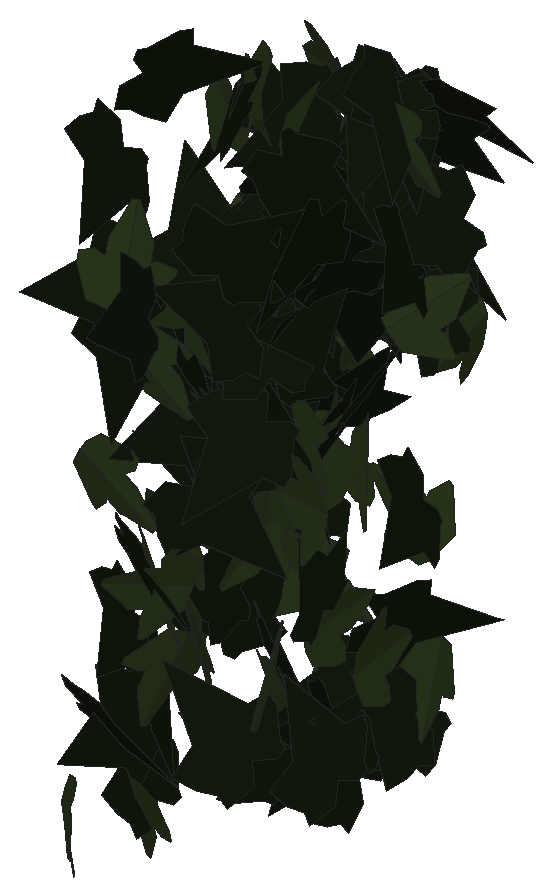
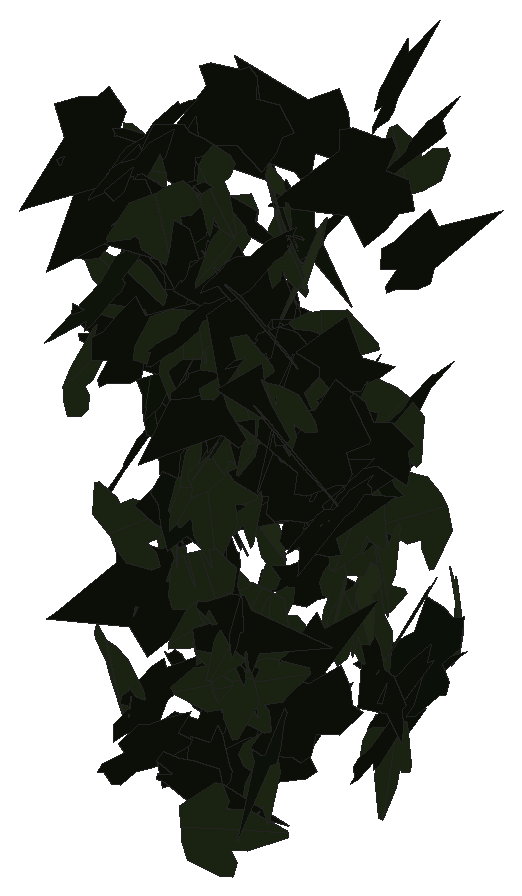
# SketchUp Ruby script. Lengths in inches.
U = 1.inch
M = Sketchup.active_model
def pt(a) = Geom::Point3d.new(a.map { |v| v * U })
def face(e, loops, mat)
  f = e.add_face(loops[0].map { |a| pt(a) })
  loops[1..].each { |l| e.add_face(l.map { |a| pt(a) }).erase! }
  f.material = f.back_material = mat if mat
  f
end
# faces: each face lists its corners as indices into pts; further lists are holes
def faces(e, pts, list, mat = nil) = list.each { |f| face(e, (f[0].is_a?(Array) ? f : [f]).map { |l| l.map { |i| pts[i] } }, mat) }
# xy, xz, yz: faces in a plane at the given z, y or x. An outline is a flat list of corners, or four numbers for a rectangle; further outlines are holes
def ring(l) = l.size == 4 ? [[l[0], l[1]], [l[2], l[1]], [l[2], l[3]], [l[0], l[3]]] : l.each_slice(2).to_a
def flat(e, list, mat, &to3) = list.each { |f| face(e, (f[0].is_a?(Array) ? f : [f]).map { |l| ring(l).map { |u, v| to3.(u, v) } }, mat) }
def xy(e, z, list, mat = nil) = flat(e, list, mat) { |x, y| [x, y, z] }
def xz(e, y, list, mat = nil) = flat(e, list, mat) { |x, z| [x, y, z] }
def yz(e, x, list, mat = nil) = flat(e, list, mat) { |y, z| [x, y, z] }
def lines(e, pts, list) = list.each { |a, b| e.add_line(pt(pts[a]), pt(pts[b])) }
# prism: a flat outline (further loops are holes) pulled along v
def prism(e, loops, v, mat = nil)
  f = face(e, loops, mat); d = Geom::Vector3d.new(v.map { |x| x * U })
  f.pushpull(f.normal.samedirection?(d) ? d.length : -d.length)
end
def box(e, o, s, mat = nil) = prism(e, [[o, [o[0] + s[0], o[1], o[2]], [o[0] + s[0], o[1] + s[1], o[2]], [o[0], o[1] + s[1], o[2]]]], [0, 0, s[2]], mat)
def at(x, y, z, deg = 0) = Geom::Transformation.translation(pt([x, y, z])) * Geom::Transformation.rotation(ORIGIN, Z_AXIS, deg.degrees)
def axes(o, x, y, z) = Geom::Transformation.new([*x, 0, *y, 0, *z, 0, *pt(o).to_a, 1])
def part(name) = M.definitions.add(name)
# library, detail: a bought-in or finely detailed component or shape, given as its bounding box
def library(name, o, s) = part(name).tap { |d| box(d.entities, o, s) }
def detail(e, o, s) = box(e.add_group.entities, o, s)
def put(e, d, t, mat = nil) = e.add_instance(d, t).tap { |i| i.material = mat if mat }
def group(e, t, mat = nil) = e.add_group.tap { |g| g.transformation = t; g.material = mat if mat }.entities
root = M.entities
M.materials.add("efeu1").color = [18, 25, 13]
M.materials.add("efeu2").color = [43, 57, 29]
c1 = part("ivyleaf_9")
p = [[1.54,2.16,1.25],[1.36,2.04,1.19],[-0.21,0.99,0.68],[-0.71,1.11,0.82],[-0.85,0.86,0.67],[-0.8,0.17,0.21],
  [-0.9,-0.01,0.1],[-0.67,-0.16,-0.02],[-0.08,-0.08,-0.05],[-0.03,-0.6,-0.4],[0.65,-0.88,-0.66],[0.83,-0.6,-0.49],
  [1.29,-0.42,-0.43],[1.8125,-0.07,-0.26],[1.21,0.44,0.15]]
faces(c1.entities,p,[[0,1,2,3,4,5,6,7,8,9,10,11,12,13,14]],"efeu1")
c2 = part("ivyleaf_10")
p = [[0,0.5,-0.03],[-0.0625,2.02,-0.43],[-0.19,2.01,-0.46],[-0.54,1.05,-0.29],[-0.52,0.625,-0.18],[-0.83,0.76,-0.28],
  [-1.16,0.64,-0.33],[-1.15,0.33,-0.24],[-0.77,-0.39,0.02],[-0.3,-0.51,0.16],[0.04,-0.48,0.23],[-0.02,2.01,-0.4375],
  [-0.06,2.01,-0.43],[0.04,-0.49,0.23],[0.67,-0.49,0.14],[1.38,0.36,-0.2],[1.375,0.51,-0.24],[0.81,0.65,-0.19],
  [0.62,0.59,-0.15],[0.6,1.09,-0.28],[0.5,1.23,-0.31]]
faces(c2.entities,p,[[0,1,2,3,4,5,6,7,8,9,10],[11,12,0,13,14,15,16,17,18,19,20]],"efeu2")
put(root,c1,axes([52.25,217.93,221.68],[-0.05075,-0.13699,0.47818],[-0.12594,-0.46146,-0.14557],[0.48121,-0.13522,0.01233]))
put(root,c2,axes([51.13,217.92,214.84],[-0.0102,0.01905,-0.49953],[0.22698,-0.44499,-0.0216],[-0.44539,-0.22721,0.00043]))
put(root,c2,axes([51.17,218.83,221.32],[0.2368,0.40848,-0.16453],[0.08062,0.14344,0.47215],[0.43293,-0.25014,0.00207]))
put(root,c1,axes([52.59,219.37,215.44],[-0.32768,-0.37509,-0.04394],[-0.02902,-0.03299,0.49807],[-0.37654,0.32896,-0.00015]))
put(root,c1,axes([50.58,219.68,220.76],[-0.1492,-0.11801,0.4624],[-0.32053,-0.33415,-0.1887],[0.35355,-0.35273,0.02406]))
put(root,c1,axes([50.24,219.4,215.24],[0.36828,-0.22379,0.25354],[0.22278,-0.12149,-0.43083],[0.25443,0.4303,0.01023]))
put(root,c1,axes([50.43,219.76,222.44],[-0.05996,-0.41817,0.26747],[-0.03648,-0.26497,-0.42245],[0.49505,-0.07018,0.00126]))
put(root,c1,axes([52.24,219.35,221.66],[-0.1215,-0.01743,0.4847],[0.46596,-0.14288,0.11166],[0.13462,0.47883,0.05096]))
put(root,c1,axes([50.73,219.52,217.54],[0.43208,-0.20442,-0.14669],[-0.13039,0.06738,-0.47797],[0.21519,0.4513,0.00491]))
put(root,c2,axes([51.09,219.95,216.88],[-0.14081,-0.09889,-0.46946],[-0.26462,-0.3921,0.16197],[-0.40018,0.29407,0.05809]))
put(root,c1,axes([50.5,220.03,214.89],[-0.14103,-0.24196,0.41421],[-0.17159,-0.37773,-0.27907],[0.44796,-0.22086,0.0235]))
put(root,c2,axes([52.625,219.58,216],[0.23907,-0.31924,0.30155],[-0.18248,0.24007,0.39883],[-0.39943,-0.30075,-0.00172]))
put(root,c1,axes([51.95,220.09,220.54],[0.05866,-0.47673,-0.13887],[0.01816,-0.13768,0.48033],[-0.49621,-0.0614,0.00116]))
put(root,c2,axes([50.73,219.71,214.18],[-0.44327,0.19916,0.11769],[-0.10581,0.05164,-0.48594],[-0.20572,-0.45571,-0.00363]))
put(root,c2,axes([51,220.08,215.98],[-0.08545,-0.45152,0.19705],[-0.01764,-0.19706,-0.45919],[0.49233,-0.08543,0.01774]))
put(root,c1,axes([50.12,220.36,216],[-0.03885,-0.30869,0.39141],[0.00307,-0.39274,-0.30943],[0.49848,-0.02163,0.03241]))
put(root,c1,axes([50.73,220,214.01],[-0.12055,-0.43794,0.20899],[0.06163,0.19978,0.45419],[-0.48132,0.13526,0.00581]))
put(root,c1,axes([53,220.18,222.23],[-0.0923,0.2247,-0.43702],[0.18885,-0.3943,-0.24262],[-0.45367,-0.20985,-0.01208]))
put(root,c1,axes([51.35,219.98,218.21],[-0.0338,-0.1462,-0.47695],[0.19794,0.43487,-0.14733],[0.4579,-0.19878,0.02848]))
put(root,c2,axes([49.74,220.21,217.9],[-0.27428,0.08199,-0.40994],[0.38793,-0.13282,-0.28612],[-0.15581,-0.47501,0.00925]))
put(root,c1,axes([50.33,220.36,215.52],[-0.15855,-0.03336,-0.47302],[0.47069,0.04945,-0.16126],[0.05754,-0.49643,0.01572]))
put(root,c2,axes([51.19,220.17,216.31],[-0.34414,0.36112,-0.03405],[0.02139,-0.02665,-0.49883],[-0.36209,-0.34479,0.0029]))
put(root,c2,axes([50.18,220.46,216.85],[-0.11885,0.0154,0.48542],[0.42602,-0.23666,0.11181],[0.2332,0.44018,0.04314]))
put(root,c2,axes([50.84,220.2,217.64],[-0.48213,0.1028,-0.08356],[0.08293,-0.01175,-0.49293],[-0.10332,-0.48918,-0.00572]))
put(root,c1,axes([51.88,220.52,219.03],[-0.44839,-0.22096,0.01116],[-0.00958,-0.0058,-0.49987],[0.22103,-0.44849,0.00097]))
put(root,c2,axes([52.94,220.13,218.47],[0.10992,-0.10806,-0.47565],[-0.36318,0.30734,-0.15375],[0.3256,0.37929,-0.01092]))
put(root,c1,axes([49.8,220.63,219.45],[0.01371,-0.47099,0.16728],[0.00304,-0.16727,-0.47118],[0.4998,0.01394,-0.00172]))
put(root,c2,axes([50.93,220.04,216.19],[0.12633,0.06004,-0.48004],[-0.26803,0.42172,-0.01779],[0.40274,0.26182,0.13874]))
put(root,c1,axes([52.35,220.375,222.72],[-0.02827,-0.02411,-0.49862],[0.33873,0.36592,-0.0369],[0.36669,-0.33988,-0.00435]))
put(root,c1,axes([53.03,220.42,214.88],[-0.4542,-0.02889,-0.20704],[-0.20675,-0.01123,0.45512],[-0.03094,0.49904,-0.00174]))
put(root,c1,axes([52.08,220.43,219.82],[-0.48137,-0.02435,0.13301],[0.13306,0.00211,0.48196],[-0.02403,0.4994,0.00445]))
put(root,c1,axes([52.07,220.54,219.79],[-0.21778,0.05231,0.44703],[0.41707,-0.16324,0.22228],[0.1692,0.4697,0.02747]))
put(root,c2,axes([50.01,220.58,219.34],[-0.41428,-0.03583,-0.27764],[0.27813,0.00379,-0.41549],[0.03187,-0.4987,0.01679]))
put(root,c1,axes([52.86,220.39,217.04],[-0.09278,0.25231,0.42158],[-0.18306,0.38039,-0.26794],[-0.45594,-0.20407,0.02178]))
put(root,c2,axes([50.97,220.77,220.17],[-0.31494,-0.38834,-0.00286],[0.00035,0.0034,-0.49999],[0.38835,-0.31493,-0.00187]))
put(root,c1,axes([51.67,221.1,214.1875],[0.0692,0.00233,0.49518],[-0.47479,-0.14172,0.06701],[0.14067,-0.47949,-0.0174]))
put(root,c1,axes([50.46,221.31,218.24],[-0.17956,-0.22396,0.40939],[-0.23974,-0.33206,-0.28681],[0.40035,-0.2993,0.01187]))
put(root,c1,axes([52.98,220.86,214.66],[-0.31892,-0.0114,-0.38492],[-0.38431,-0.02235,0.31907],[-0.02448,0.49937,0.00549]))
put(root,c1,axes([52.57,221.08,220.78],[0.2722,0.32868,0.26052],[-0.1671,-0.19988,0.42676],[0.38468,-0.3194,0.00103]))
put(root,c1,axes([51.16,221.16,217.64],[-0.09333,0.01584,0.49096],[-0.49015,0.02983,-0.09414],[-0.03228,-0.49886,0.00996]))
put(root,c1,axes([52.31,220.73,220.62],[0.02613,0.46386,0.18481],[0.01491,0.18426,-0.46457],[-0.49909,0.02979,-0.0042]))
put(root,c1,axes([50.48,221.16,219.02],[0.06662,-0.41695,0.26779],[-0.04298,0.26432,0.42224],[-0.49367,-0.07928,-0.00062]))
put(root,c1,axes([53.17,221.58,221.25],[0.00819,-0.28542,0.41045],[0.01659,-0.41012,-0.28553],[0.49966,0.01829,0.00275]))
put(root,c1,axes([50.61,221.15,218.54],[0.4822,-0.12266,0.04942],[0.0485,-0.00981,-0.49755],[0.12303,0.48462,0.00244]))
put(root,c1,axes([49.95,220.87,222.79],[0.0406,0.22589,-0.44421],[0.02619,0.4441,0.22823],[0.49766,-0.04179,0.02423]))
put(root,c2,axes([53.16,220.88,216.13],[0.0089,-0.00005,0.49992],[-0.2007,0.45794,0.00362],[-0.45787,-0.20073,0.00813]))
put(root,c1,axes([51.51,221.55,218.28],[0.23566,-0.43888,-0.04297],[0.03235,-0.03138,0.49796],[-0.43979,-0.23749,0.01361]))
put(root,c1,axes([50.59,221.68,215.96],[-0.06813,-0.10168,0.48479],[-0.26431,-0.4064,-0.12238],[0.41892,-0.27295,0.00163]))
put(root,c2,axes([50.57,221.68,219.78],[-0.02864,-0.16214,-0.47211],[-0.07156,-0.46667,0.16461],[-0.49402,0.07699,0.00353]))
put(root,c1,axes([53.24,221.72,217.97],[-0.03509,-0.31856,0.38378],[-0.03025,-0.38266,-0.3204],[0.49785,-0.04571,0.00758]))
put(root,c1,axes([50.23,221.45,218.26],[0.13945,-0.45793,-0.14442],[-0.0396,0.1389,-0.47868],[0.47852,0.14494,0.00247]))
put(root,c1,axes([52,221.09,220.65],[-0.05588,0.46651,0.17101],[-0.01665,0.17023,-0.46983],[-0.49659,-0.0582,-0.00349]))
put(root,c1,axes([52.87,221.3,220.69],[0.09503,0.45393,-0.18686],[-0.05732,-0.17877,-0.46342],[-0.48753,0.1095,0.01806]))
put(root,c1,axes([49.65,221.45,219.66],[-0.1611,-0.15811,-0.44615],[0.36132,0.26337,-0.2238],[0.30577,-0.39451,0.0294]))
put(root,c1,axes([52.1875,221.5625,214.66],[0.04885,0.25549,-0.42701],[-0.10455,-0.41422,-0.25979],[-0.4865,0.11467,0.01295]))
put(root,c1,axes([50.76,221.61,222.35],[-0.38642,0.27952,-0.15016],[0.11605,-0.09572,-0.47683],[-0.29531,-0.40337,0.0091]))
put(root,c1,axes([50.37,221.52,220.125],[-0.44695,-0.1928,0.11429],[0.10464,0.04595,0.48676],[-0.1982,0.45904,-0.00073]))
put(root,c1,axes([52.85,222.02,214.9],[0.02718,-0.38108,-0.32255],[0.08235,-0.31519,0.37931],[-0.49242,-0.07374,0.04563]))
put(root,c2,axes([52.14,221.29,216.1],[0.04574,-0.02935,0.49704],[-0.13103,0.48083,0.04045],[-0.48035,-0.13396,0.03629]))
put(root,c1,axes([51.31,221.98,218.83],[-0.19195,-0.05484,0.45842],[-0.43256,-0.15218,-0.19933],[0.16138,-0.47311,0.01098]))
put(root,c1,axes([50.87,221.83,218.42],[-0.05443,0.0653,0.49272],[-0.49602,0.02435,-0.05802],[-0.03157,-0.49512,0.06213]))
put(root,c2,axes([53.04,221.68,220.33],[0.32055,0.00149,-0.38372],[0.38326,0.02333,0.32026],[0.01886,-0.49945,0.01381]))
put(root,c2,axes([51.29,221.84,218.375],[-0.37448,0.21153,-0.25499],[0.21086,-0.14466,-0.42967],[-0.25555,-0.42933,0.01914]))
put(root,c2,axes([50.76,222.1,216.69],[0.03167,0.26665,-0.42177],[-0.11359,-0.40767,-0.26627],[-0.48589,0.11269,0.03475]))
put(root,c2,axes([50.8,221.875,222.64],[0.30888,-0.39256,-0.02217],[-0.01272,0.0182,-0.49951],[0.39298,0.30914,0.00125]))
put(root,c1,axes([50.92,222.12,220.57],[-0.24978,-0.43313,0.00249],[-0.00114,-0.00222,-0.49999],[0.43314,-0.24978,0.00012]))
put(root,c2,axes([51.375,222.06,220.78],[-0.09784,-0.45076,0.19299],[-0.04289,-0.18817,-0.46125],[0.48845,-0.10681,-0.00184]))
put(root,c1,axes([52.83,221.54,216.38],[0.02184,0.20788,-0.45421],[0.07276,0.44847,0.20875],[0.49419,-0.07522,-0.01066]))
put(root,c2,axes([52.6,222.04,222.4],[-0.15595,0.11334,-0.46134],[0.38981,-0.247,-0.19246],[-0.27153,-0.4197,-0.01132]))
put(root,c1,axes([50.33,221.73,215.3],[-0.12036,-0.07804,0.47898],[0.46177,0.13338,0.13776],[-0.14927,0.47552,0.03997]))
put(root,c1,axes([51.625,222.07,222.33],[-0.48214,0.03505,0.12773],[-0.12856,-0.00783,-0.48313],[-0.03187,-0.49871,0.01656]))
put(root,c1,axes([52.51,222.16,222.95],[-0.37194,-0.31893,-0.09973],[0.08414,0.05503,-0.48979],[0.32339,-0.38113,0.01273]))
put(root,c1,axes([52.53,222.23,222.97],[0.01382,-0.49343,0.0796],[-0.01152,-0.07992,-0.49344],[0.49968,0.0118,-0.01357]))
put(root,c1,axes([52.54,222.31,221.97],[-0.15551,-0.45169,0.14761],[0.02171,-0.16191,-0.47256],[0.47471,-0.14057,0.06997]))
put(root,c2,axes([50.16,221.875,222.15],[0.24821,-0.4258,-0.08421],[0.2118,0.20349,-0.40464],[0.37886,0.1652,0.28138]))
put(root,c1,axes([53.27,222.36,221.39],[-0.25937,-0.21359,0.37028],[-0.21788,-0.30657,-0.32946],[0.36777,-0.33226,0.06595]))
put(root,c1,axes([52.46,221.875,219.22],[-0.25593,0.42875,-0.02593],[0.01144,-0.02337,-0.49932],[-0.42938,-0.25618,0.00215]))
put(root,c2,axes([50.79,221.83,222.09],[-0.1357,0.04471,0.47915],[-0.45826,0.13997,-0.14285],[-0.14691,-0.47792,0.00299]))
put(root,c2,axes([50.84,221.71,219.67],[-0.0289,0.36118,0.34454],[-0.04633,0.34169,-0.36208],[-0.49701,-0.05285,0.01372]))
put(root,c2,axes([50.83,222.01,214.73],[-0.38179,0.28748,-0.14693],[0.12008,-0.08478,-0.4779],[-0.29969,-0.40021,-0.00431]))
put(root,c1,axes([49.875,221.74,219.34],[0.06938,0.02472,0.49455],[0.43676,0.23223,-0.07288],[-0.2333,0.44211,0.01063]))
put(root,c1,axes([51.41,222.22,214.3],[0.266,-0.09692,-0.41213],[0.42184,0.01922,0.26774],[-0.03606,-0.49014,0.092]))
put(root,c1,axes([51.41,221.97,221.25],[-0.31588,0.3243,0.21224],[-0.17394,0.12606,-0.4515],[-0.34636,-0.35908,0.03317]))
put(root,c1,axes([50.53,221.875,220.21],[0.17605,-0.12267,-0.45162],[-0.37112,0.25736,-0.21457],[0.2851,0.41075,-0.00044]))
put(root,c1,axes([51.95,222.4375,219.89],[0.35344,-0.25173,-0.24842],[0.20137,-0.14549,0.43392],[-0.29075,-0.40677,-0.00146]))
put(root,c2,axes([53,222.12,217.29],[0.30725,0.06587,0.38892],[-0.37936,-0.08573,0.31422],[0.10808,-0.48817,-0.00271]))
put(root,c2,axes([53.01,222.24,215.63],[0.4494,-0.20646,0.07357],[0.06733,-0.02968,-0.49456],[0.20858,0.45442,0.00113]))
put(root,c1,axes([51.16,221.95,221.43],[0.30604,0.37392,-0.12856],[-0.08632,-0.09546,-0.48315],[-0.38586,0.31792,0.00613]))
put(root,c1,axes([51.27,222.53,219.16],[0.27139,-0.33525,-0.2529],[0.15726,-0.19807,0.43132],[-0.38938,-0.31365,-0.00207]))
put(root,c2,axes([51.36,221.81,221.98],[-0.04962,0.16868,0.46807],[-0.13038,0.44954,-0.17583],[-0.48014,-0.1395,-0.00063]))
put(root,c2,axes([51.36,222.35,218.93],[0.11443,0.40965,-0.26285],[-0.08258,-0.24976,-0.42521],[-0.47967,0.14073,0.0105]))
put(root,c1,axes([50.68,222.03,215.37],[0.33247,-0.07766,-0.36528],[-0.34198,0.13317,-0.33958],[0.15004,0.47564,0.03544]))
put(root,c1,axes([52.48,222.6,214.62],[-0.24738,-0.34044,0.27001],[-0.16623,-0.21291,-0.42076],[0.40146,-0.29794,-0.00785]))
put(root,c2,axes([51.05,222.35,215.96],[-0.15165,-0.0165,-0.47616],[-0.47406,-0.04475,0.15253],[-0.04765,0.49772,-0.00207]))
put(root,c1,axes([52.46,222.48,222.79],[0.0034,-0.49706,-0.05404],[-0.00051,0.05404,-0.49707],[0.49999,0.00344,-0.00014]))
put(root,c1,axes([53.19,222.37,220.07],[-0.39151,0.10486,0.29279],[-0.28662,0.06103,-0.40512],[-0.1207,-0.48506,0.01232]))
put(root,c1,axes([51.48,222.31,218.27],[0.36518,0.33398,0.07143],[-0.05345,-0.04739,0.49487],[0.33732,-0.36907,0.00109]))
put(root,c1,axes([51.09,222.53,220.32],[-0.17902,-0.45288,-0.11336],[0.06438,0.0963,-0.4864],[0.46239,-0.18875,0.02383]))
put(root,c1,axes([52.03,222.37,222.0625],[-0.03313,-0.02268,-0.49839],[0.46423,0.18156,-0.03912],[0.18275,-0.46532,0.00903]))
put(root,c2,axes([51.72,222.55,217.86],[0.29304,-0.23531,0.32979],[0.28952,-0.16307,-0.37361],[0.28339,0.40992,0.04068]))
put(root,c2,axes([51.42,222.41,218.6],[-0.23876,-0.43843,0.02785],[-0.01534,-0.02335,-0.49922],[0.43904,-0.23924,-0.0023]))
put(root,c1,axes([50.62,222.54,222.12],[0.00207,-0.49075,-0.09571],[0.02773,0.09568,-0.48998],[0.49923,-0.00328,0.02762]))
put(root,c1,axes([50.29,222.02,220.14],[0.10627,0.07598,0.48263],[0.2619,0.4081,-0.12192],[-0.41245,0.27871,0.04693]))
put(root,c1,axes([51.57,222.76,220.84],[-0.13839,-0.44322,0.18548],[-0.04549,-0.18006,-0.46423],[0.47831,-0.14536,0.00951]))
put(root,c2,axes([50.99,222.43,216.06],[-0.24033,0.0412,-0.43651],[0.42673,-0.09237,-0.24366],[-0.10072,-0.48966,0.00924]))
put(root,c2,axes([50.84,222.25,217.05],[-0.21641,-0.34542,-0.28957],[0.16835,0.23603,-0.40737],[0.41812,-0.27382,0.01414]))
put(root,c2,axes([51.78,222.4375,220.63],[-0.41927,-0.27226,0.00955],[0.01161,-0.03537,-0.49861],[0.27218,-0.41788,0.03598]))
put(root,c1,axes([51.72,222.54,218.6],[-0.23688,0.3189,-0.30363],[0.1661,-0.25459,-0.39698],[-0.4078,-0.28894,0.01467]))
put(root,c1,axes([51.72,222.59,214.55],[-0.43634,0.03121,0.24215],[-0.24342,-0.0172,-0.43641],[-0.01892,-0.49873,0.0302]))
put(root,c2,axes([51.52,222.23,222.75],[0.14914,-0.02865,-0.47638],[-0.32979,0.35457,-0.12457],[0.34496,0.35137,0.08687]))
put(root,c2,axes([50.31,222.52,220.28],[0.49882,-0.00567,0.03386],[0.03389,0.00301,-0.49884],[0.00545,0.49996,0.00339]))
put(root,c1,axes([50.77,222.66,217.54],[-0.01018,0.00509,-0.49987],[0.49692,-0.05438,-0.01067],[-0.05448,-0.49701,-0.00395]))
put(root,c2,axes([51.47,222.79,218.76],[-0.02627,0.26016,-0.42618],[0.00794,-0.4265,-0.26084],[-0.49925,-0.02047,0.01828]))
put(root,c2,axes([51.22,222.75,214.04],[0.0229,0.01091,0.49936],[-0.34613,-0.36005,0.02374],[0.3601,-0.34677,-0.00893]))
put(root,c2,axes([50.98,222.49,220.54],[-0.42909,-0.01695,0.25611],[-0.25548,-0.01968,-0.42935],[0.02464,-0.49932,0.00823]))
put(root,c1,axes([52.48,222.91,220.24],[-0.1033,-0.13226,0.471],[-0.32431,-0.34189,-0.16713],[0.36626,-0.34003,-0.01515]))
put(root,c2,axes([53.06,222.9,219.7],[-0.07384,-0.01356,0.49433],[0.23569,-0.44036,0.02312],[0.43474,0.23643,0.07142]))
put(root,c1,axes([51.02,222.73,216.96],[-0.18362,-0.18565,-0.4264],[-0.28585,-0.31656,0.26092],[-0.36684,0.3396,0.01011]))
put(root,c2,axes([51.35,222.59,217.51],[-0.4436,-0.03672,0.22775],[-0.21436,-0.11681,-0.43636],[0.08525,-0.48478,0.08789]))
put(root,c2,axes([52.04,222.6,222.35],[0.23453,0.42623,-0.11543],[-0.08357,-0.0855,-0.4855],[-0.4336,0.24702,0.03113]))
put(root,c1,axes([52.92,222.36,222.88],[0.49031,0.06883,0.06973],[0.0659,0.03166,-0.49463],[-0.0725,0.49423,0.02198]))
put(root,c1,axes([50.43,222.4375,219.78],[-0.30232,0.28906,0.27395],[-0.21364,0.17255,-0.41783],[-0.3361,-0.36969,0.01918]))
put(root,c1,axes([51.15,222.34,220.07],[0.45547,0.18589,0.0894],[0.08486,0.02866,-0.49191],[-0.18801,0.46328,-0.00544]))
put(root,c1,axes([52.66,222.58,221.09],[0.37156,-0.31965,-0.09884],[-0.01993,0.1263,-0.48338],[0.33399,0.36314,0.08112]))
put(root,c1,axes([52.67,222.37,222.37],[0.42602,0.25295,0.06728],[0.0639,0.02412,-0.49531],[-0.25382,0.43062,-0.01177]))
